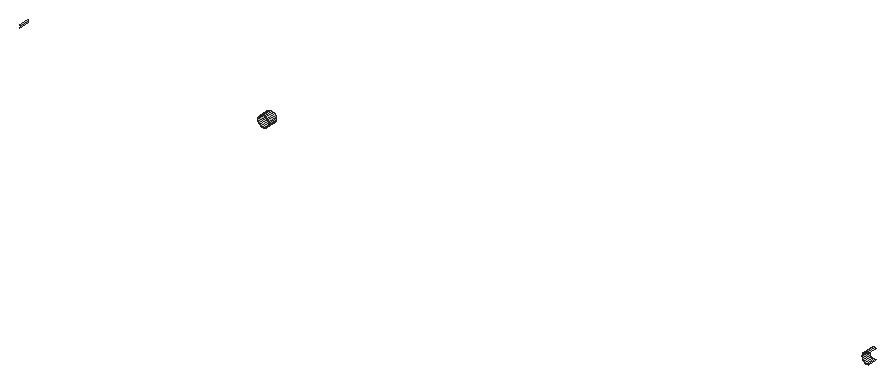
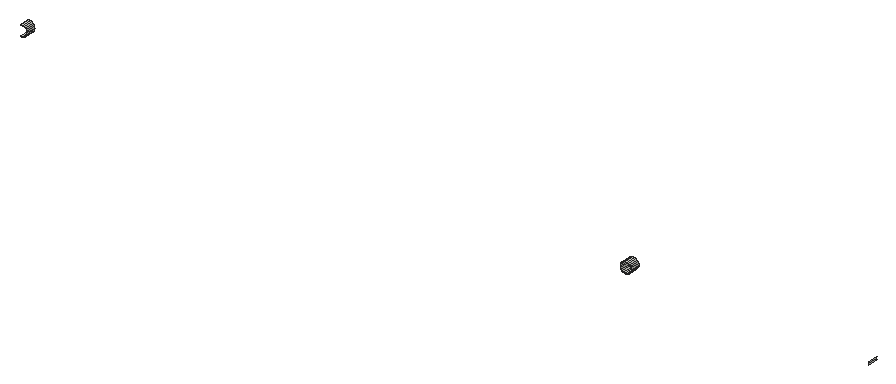
# SketchUp Ruby script. Lengths in inches.
U = 1.inch
M = Sketchup.active_model
def pt(a) = Geom::Point3d.new(a.map { |v| v * U })
def face(e, loops, mat)
  f = e.add_face(loops[0].map { |a| pt(a) })
  loops[1..].each { |l| e.add_face(l.map { |a| pt(a) }).erase! }
  f.material = f.back_material = mat if mat
  f
end
# faces: each face lists its corners as indices into pts; further lists are holes
def faces(e, pts, list, mat = nil) = list.each { |f| face(e, (f[0].is_a?(Array) ? f : [f]).map { |l| l.map { |i| pts[i] } }, mat) }
# xy, xz, yz: faces in a plane at the given z, y or x. An outline is a flat list of corners, or four numbers for a rectangle; further outlines are holes
def ring(l) = l.size == 4 ? [[l[0], l[1]], [l[2], l[1]], [l[2], l[3]], [l[0], l[3]]] : l.each_slice(2).to_a
def flat(e, list, mat, &to3) = list.each { |f| face(e, (f[0].is_a?(Array) ? f : [f]).map { |l| ring(l).map { |u, v| to3.(u, v) } }, mat) }
def xy(e, z, list, mat = nil) = flat(e, list, mat) { |x, y| [x, y, z] }
def xz(e, y, list, mat = nil) = flat(e, list, mat) { |x, z| [x, y, z] }
def yz(e, x, list, mat = nil) = flat(e, list, mat) { |y, z| [x, y, z] }
def lines(e, pts, list) = list.each { |a, b| e.add_line(pt(pts[a]), pt(pts[b])) }
# prism: a flat outline (further loops are holes) pulled along v
def prism(e, loops, v, mat = nil)
  f = face(e, loops, mat); d = Geom::Vector3d.new(v.map { |x| x * U })
  f.pushpull(f.normal.samedirection?(d) ? d.length : -d.length)
end
def box(e, o, s, mat = nil) = prism(e, [[o, [o[0] + s[0], o[1], o[2]], [o[0] + s[0], o[1] + s[1], o[2]], [o[0], o[1] + s[1], o[2]]]], [0, 0, s[2]], mat)
def at(x, y, z, deg = 0) = Geom::Transformation.translation(pt([x, y, z])) * Geom::Transformation.rotation(ORIGIN, Z_AXIS, deg.degrees)
def axes(o, x, y, z) = Geom::Transformation.new([*x, 0, *y, 0, *z, 0, *pt(o).to_a, 1])
def part(name) = M.definitions.add(name)
# library, detail: a bought-in or finely detailed component or shape, given as its bounding box
def library(name, o, s) = part(name).tap { |d| box(d.entities, o, s) }
def detail(e, o, s) = box(e.add_group.entities, o, s)
def put(e, d, t, mat = nil) = e.add_instance(d, t).tap { |i| i.material = mat if mat }
def group(e, t, mat = nil) = e.add_group.tap { |g| g.transformation = t; g.material = mat if mat }.entities
root = M.entities
p = [[2663.06,801.78,132.03],[2663.33,801.78,131.92],[2663.33,799.91,131.92],[2663.06,799.91,132.03],[2663.62,801.78,131.88],[2663.62,799.91,131.88],
  [2663.91,801.78,131.92],[2663.91,799.91,131.92],[2664.18,801.78,132.03],[2664.18,799.91,132.03],[2787.4,801.78,132.03],[2787.67,801.78,131.92],
  [2787.67,799.91,131.92],[2787.4,799.91,132.03],[2787.96,801.78,131.88],[2787.96,799.91,131.88],[2788.25,801.78,131.92],[2788.25,799.91,131.92],
  [2662.83,801.78,132.21],[2662.83,799.91,132.21],[2664.42,801.78,132.21],[2664.42,799.91,132.21],[2787.17,801.78,132.21],[2787.17,799.91,132.21],
  [2662.65,801.78,132.44],[2662.65,799.91,132.44],[2664.6,801.78,132.44],[2664.6,799.91,132.44],[2786.99,801.78,132.44],[2786.99,799.91,132.44],
  [2662.53,801.78,132.71],[2662.53,799.91,132.71],[2664.71,801.78,132.71],[2664.71,799.91,132.71],[2786.875,801.78,132.71],[2786.875,799.91,132.71],
  [2613.58,801.78,132.71],[2613.62,801.78,133],[2613.62,799.91,133],[2613.58,799.91,132.71],[2662.5,801.78,133],[2662.5,799.91,133],
  [2664.75,801.78,133],[2664.75,799.91,133],[2786.84,801.78,133],[2786.84,799.91,133],[2613.58,801.78,133.29],[2613.58,799.91,133.29],
  [2662.53,801.78,133.29],[2662.53,799.91,133.29],[2664.71,801.78,133.29],[2664.71,799.91,133.29],[2786.875,801.78,133.29],[2786.875,799.91,133.29],
  [2662.65,801.78,133.57],[2662.65,799.91,133.57],[2664.6,801.78,133.57],[2664.6,799.91,133.57],[2786.99,801.78,133.57],[2786.99,799.91,133.57],
  [2662.83,801.78,133.8],[2662.83,799.91,133.8],[2664.42,801.78,133.8],[2664.42,799.91,133.8],[2787.17,801.78,133.8],[2787.17,799.91,133.8],
  [2663.06,801.78,133.98],[2663.06,799.91,133.98],[2664.18,801.78,133.98],[2664.18,799.91,133.98],[2787.4,801.78,133.98],[2787.4,799.91,133.98],
  [2663.33,801.78,134.09],[2663.33,799.91,134.09],[2663.91,801.78,134.09],[2663.91,799.91,134.09],[2787.67,801.78,134.09],[2787.67,799.91,134.09],
  [2663.62,801.78,134.13],[2663.62,799.91,134.13],[2787.96,801.78,134.13],[2787.96,799.91,134.13],[2788.25,801.78,134.09],[2788.25,799.91,134.09]]
faces(root,p,[[0,1,2,3],[1,4,5,2],[4,6,7,5],[6,8,9,7],[10,11,12,13],[11,14,15,12],[14,16,17,15],[18,0,3,19],
  [8,20,21,9],[22,10,13,23],[24,18,19,25],[20,26,27,21],[28,22,23,29],[30,24,25,31],[26,32,33,27],[34,28,29,35],
  [36,37,38,39],[40,30,31,41],[32,42,43,33],[44,34,35,45],[37,46,47,38],[48,40,41,49],[42,50,51,43],[52,44,45,53],
  [54,48,49,55],[50,56,57,51],[58,52,53,59],[60,54,55,61],[56,62,63,57],[64,58,59,65],[66,60,61,67],[62,68,69,63],
  [70,64,65,71],[72,66,67,73],[68,74,75,69],[76,70,71,77],[78,72,73,79],[74,78,79,75],[80,76,77,81],[82,80,81,83]])
